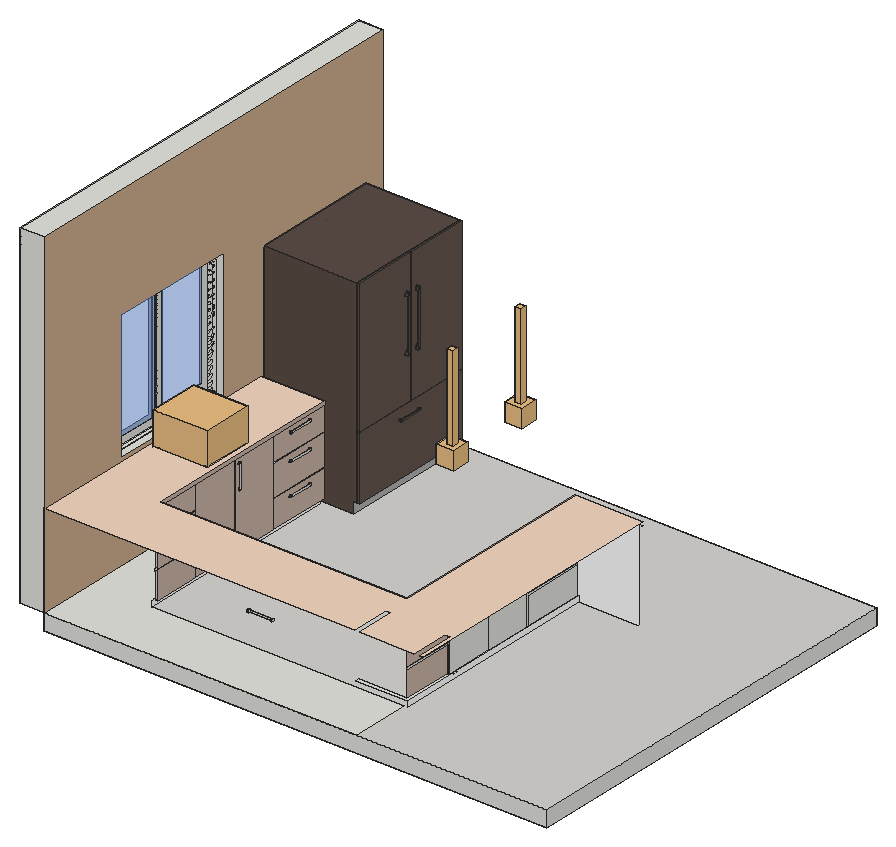
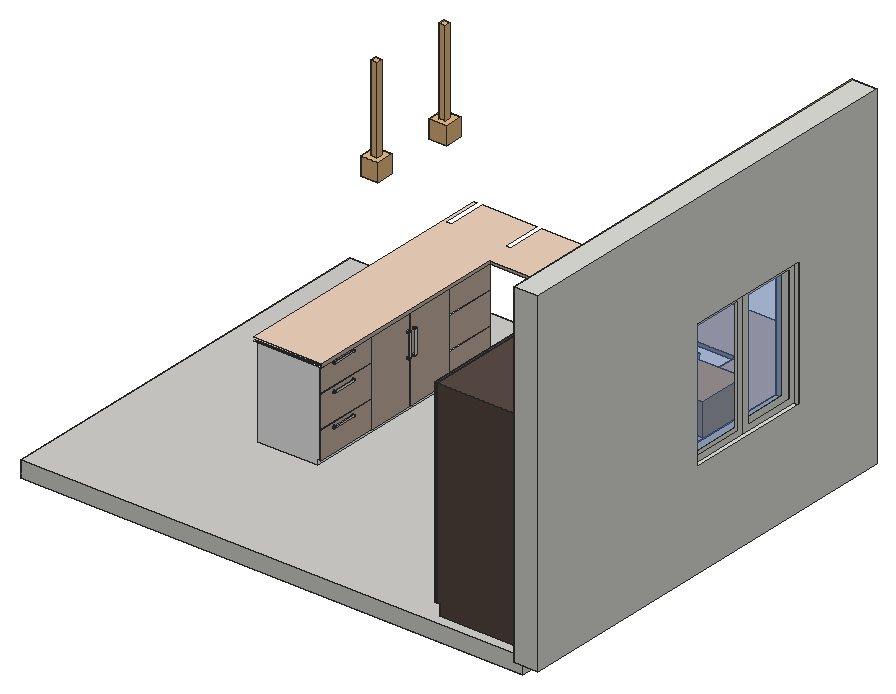
# SketchUp Ruby script. Lengths in inches.
U = 1.inch
M = Sketchup.active_model
def pt(a) = Geom::Point3d.new(a.map { |v| v * U })
def face(e, loops, mat)
  f = e.add_face(loops[0].map { |a| pt(a) })
  loops[1..].each { |l| e.add_face(l.map { |a| pt(a) }).erase! }
  f.material = f.back_material = mat if mat
  f
end
# faces: each face lists its corners as indices into pts; further lists are holes
def faces(e, pts, list, mat = nil) = list.each { |f| face(e, (f[0].is_a?(Array) ? f : [f]).map { |l| l.map { |i| pts[i] } }, mat) }
# xy, xz, yz: faces in a plane at the given z, y or x. An outline is a flat list of corners, or four numbers for a rectangle; further outlines are holes
def ring(l) = l.size == 4 ? [[l[0], l[1]], [l[2], l[1]], [l[2], l[3]], [l[0], l[3]]] : l.each_slice(2).to_a
def flat(e, list, mat, &to3) = list.each { |f| face(e, (f[0].is_a?(Array) ? f : [f]).map { |l| ring(l).map { |u, v| to3.(u, v) } }, mat) }
def xy(e, z, list, mat = nil) = flat(e, list, mat) { |x, y| [x, y, z] }
def xz(e, y, list, mat = nil) = flat(e, list, mat) { |x, z| [x, y, z] }
def yz(e, x, list, mat = nil) = flat(e, list, mat) { |y, z| [x, y, z] }
def lines(e, pts, list) = list.each { |a, b| e.add_line(pt(pts[a]), pt(pts[b])) }
# prism: a flat outline (further loops are holes) pulled along v
def prism(e, loops, v, mat = nil)
  f = face(e, loops, mat); d = Geom::Vector3d.new(v.map { |x| x * U })
  f.pushpull(f.normal.samedirection?(d) ? d.length : -d.length)
end
def box(e, o, s, mat = nil) = prism(e, [[o, [o[0] + s[0], o[1], o[2]], [o[0] + s[0], o[1] + s[1], o[2]], [o[0], o[1] + s[1], o[2]]]], [0, 0, s[2]], mat)
def at(x, y, z, deg = 0) = Geom::Transformation.translation(pt([x, y, z])) * Geom::Transformation.rotation(ORIGIN, Z_AXIS, deg.degrees)
def axes(o, x, y, z) = Geom::Transformation.new([*x, 0, *y, 0, *z, 0, *pt(o).to_a, 1])
def part(name) = M.definitions.add(name)
# library, detail: a bought-in or finely detailed component or shape, given as its bounding box
def library(name, o, s) = part(name).tap { |d| box(d.entities, o, s) }
def detail(e, o, s) = box(e.add_group.entities, o, s)
def put(e, d, t, mat = nil) = e.add_instance(d, t).tap { |i| i.material = mat if mat }
def group(e, t, mat = nil) = e.add_group.tap { |g| g.transformation = t; g.material = mat if mat }.entities
root = M.entities
M.materials.add("2").color = [91, 76, 69]
M.materials.add("Emissive\#2").color = [255, 255, 255]
M.materials.add("Emissive\#3").color = [255, 255, 255]
M.materials.add("[0008_LavenderBlush]").color = [212, 210, 207]
M.materials.add("[Aluminum]").color = [179, 179, 179]
M.materials.add("[Color A01]5").color = [206, 173, 143]
M.materials.add("[Color B01]").color = [102, 86, 78]
M.materials.add("[Color D01]").color = [201, 180, 165]
M.materials.add("[Color D02]").color = [242, 213, 191]
M.materials.add("[Translucent Glass Blue]").color = [100, 149, 237]
M.materials["[Translucent Glass Blue]"].alpha = 0.5
c1 = part("Group\#8")
prism(c1.entities,[[[0.125,0.37,0],[0.125,1.02,0],[0.125,1.04,0],[0.125,1.0625,0.01],[0.125,1.08,0.01],[0.125,1.1,0.02],[0.125,1.12,0.04],[0.125,1.14,0.05],[0.125,1.15,0.07],[0.125,1.16,0.09],[0.125,1.17,0.11],[0.125,1.18,0.125],[0.125,1.1875,0.15],[0.125,1.1875,0.17],[0.125,1.1875,3.72],[0.125,1.18,3.74],[0.125,1.18,3.76],[0.125,1.17,3.78],[0.125,1.16,3.8],[0.125,1.14,3.81],[0.125,1.125,3.83],[0.125,1.11,3.84],[0.125,1.09,3.85],[0.125,1.07,3.86],[0.125,1.05,3.87],[0.125,1.03,3.875],[0.125,1.01,3.875],[0.125,0.37,3.875],[0.125,0.37,3.625],[0.125,0.9375,3.625],[0.125,0.9375,0.25],[0.125,0.37,0.25]]],[-0.125,0,0])
c2 = part("Group\#171")
prism(c2.entities,[[[0,0.37,0],[0,0.37,0.25],[0,0.9375,0.25],[0,0.9375,3.625],[0,0.37,3.625],[0,0.37,3.875],[0,1.01,3.875],[0,1.03,3.875],[0,1.05,3.87],[0,1.07,3.86],[0,1.09,3.85],[0,1.11,3.84],[0,1.125,3.83],[0,1.14,3.81],[0,1.16,3.8],[0,1.17,3.78],[0,1.18,3.76],[0,1.18,3.74],[0,1.1875,3.72],[0,1.1875,0.17],[0,1.1875,0.15],[0,1.18,0.125],[0,1.17,0.11],[0,1.16,0.09],[0,1.15,0.07],[0,1.14,0.05],[0,1.12,0.04],[0,1.1,0.02],[0,1.08,0.01],[0,1.0625,0.01],[0,1.04,0],[0,1.02,0]]],[0.125,0,0])
c3 = library("Pendant light \#2",[-0.17,-0.17,-2.26],[2.36,2.36,34.63])
c4 = library("Sink with faucet",[-0.11,0,0],[20.3,18.9,21.51])
xy(root,6,[[8.9375,9,8.9375,110.3125,31.25,110.3125,31.25,31.3125,125.9375,31.3125,125.9375,9]])
xy(root,6,[[9,111.6875,11.8125,159.6875],[11.8125,111.6875,42.9375,159.6875]],"2")
xy(root,8,[[107.9375,31.3125,107.9375,32.625,125.9375,32.625,125.9375,51.3125,127.25,51.3125,127.25,31.3125],[31.25,32.625,31.9375,50],[31.9375,32.625,32.5625,50],[31.25,50,31.9375,50.5],[31.25,50.5,31.9375,68.5],
  [31.9375,50.5,32.5625,68.5],[126.5625,51.3125,127.25,51.8125],[125.9375,51.8125,126.5625,69.8125],[126.5625,51.8125,127.25,69.8125],[31.25,68.5,31.9375,69],
  [31.25,69,31.9375,86.5],[31.9375,69,32.5625,86.5],[125.9375,69.8125,126.5625,70.3125],[126.5625,69.8125,127.25,111.625],[125.9375,70.3125,126.5625,87.8125],
  [31.25,86.5,31.9375,86.99],[31.25,86.99,31.9375,110.3125],[31.9375,86.99,32.5625,110.3125],[125.9375,87.8125,126.5625,88.3],[125.9375,88.3,126.5625,111.625]])
xy(root,10.07,[[11.8125,111.6875,12.875,135.1875],[42.9375,111.6875,44,135.1875],[44,111.6875,45,159.6875],[11.8125,135.1875,12.875,136.1875],[42.9375,135.1875,44,136.1875],
  [42.9375,136.1875,44,159.6875]],"2")
xy(root,18.125,[[31.9375,32.625,32.5625,50],[31.9375,86.99,32.5625,110.3125],[125.9375,88.3,126.5625,111.625]])
xy(root,18.625,[[31.9375,32.625,32.5625,50],[31.9375,86.99,32.5625,110.3125],[125.9375,88.3,126.5625,111.625]])
xy(root,28.5,[[12.67,58,30.19,58,30.29,58.02,30.39,58.06,30.48,58.1,30.57,58.16,30.64,58.23,30.71,58.31,30.77,58.39,30.81,58.48,30.85,58.58,30.87,58.68,30.875,58.79,30.875,76.11,30.87,76.21,30.85,76.3125,30.81,76.41,30.77,76.5,30.71,76.59,30.57,76.73,30.48,76.79,30.39,76.84,30.29,76.87,30.19,76.89,30.09,76.9,12.76,76.9,12.66,76.89,12.5625,76.87,12.46,76.84,12.37,76.79,12.29,76.73,12.21,76.66,12.14,76.59,12.08,76.5,12.04,76.41,12,76.3125,11.98,76.21,11.98,58.68,12,58.59,12.03,58.5,12.07,58.41,12.12,58.33,12.24,58.19,12.4,58.09,12.49,58.05,12.58,58.02]])
xy(root,30.125,[[31.9375,32.625,32.5625,50],[31.9375,86.99,32.5625,110.3125],[125.9375,88.3,126.5625,111.625]])
xy(root,30.625,[[31.9375,32.625,32.5625,50],[31.9375,86.99,32.5625,110.3125],[125.9375,88.3,126.5625,111.625]])
xy(root,33.92,[[44,111.6875,45,159.6875]],"2")
xy(root,34.38,[[12.875,111.6875,13.875,135.1875],[44,111.6875,45,135.1875],[44,136.1875,45,159.6875]],"2")
xy(root,39.75,[[31.9375,32.625,32.5625,32.75],[31.9375,32.75,32.5625,50],[31.9375,50.5,32.5625,68.5],[125.9375,51.8125,126.5625,69.8125],[31.9375,69,32.5625,86.5],
  [125.9375,70.3125,126.5625,87.8125],[31.9375,86.99,32.5625,110.3125],[125.9375,88.3,126.5625,111.625]])
xy(root,39.75,[[49.9375,32,49.9375,32.625,32.5625,32.625,32.5625,32.75,32.6875,32.75,32.6875,33.25,125.3125,33.25,125.3125,112.25,150.8125,112.25,150.8125,111.625,125.9375,111.625,125.9375,88.3,126.5625,88.3,126.5625,87.8125,125.9375,87.8125,125.9375,70.3125,126.5625,70.3125,126.5625,69.8125,125.9375,69.8125,125.9375,51.8125,126.5625,51.8125,126.5625,51.3125,125.9375,51.3125,125.9375,32.625,107.9375,32.625,107.9375,32,107.4375,32,107.4375,32.625,89.4375,32.625,89.4375,32,88.9375,32,88.9375,32.625,50.4375,32.625,50.4375,32],[32.5625,32.75,32.5625,50,31.9375,50,31.9375,50.5,32.5625,50.5,32.5625,68.5,31.9375,68.5,31.9375,69,32.5625,69,32.5625,86.5,31.9375,86.5,31.9375,86.99,32.5625,86.99,32.5625,110.3125,33.1875,110.3125,33.1875,33.25,32.6875,33.25,32.6875,32.75]],"Emissive\#2")
xy(root,41,[[[8.9375,9,125.3125,9,125.3125,23.51,127.1875,23.51,127.1875,9,147.625,9,147.625,23.51,149.5625,23.51,149.5625,9,150.8125,9,150.8125,112.25,125.3125,112.25,125.3125,33.25,33.1875,33.25,33.1875,110.3125,8.9375,110.3125],[12.67,58,12.58,58.02,12.49,58.05,12.4,58.09,12.24,58.19,12.12,58.33,12.07,58.41,12.03,58.5,12,58.59,11.98,58.68,11.98,76.21,12,76.3125,12.04,76.41,12.08,76.5,12.14,76.59,12.21,76.66,12.29,76.73,12.37,76.79,12.46,76.84,12.5625,76.87,12.66,76.89,12.76,76.9,30.09,76.9,30.19,76.89,30.29,76.87,30.39,76.84,30.48,76.79,30.57,76.73,30.71,76.59,30.77,76.5,30.81,76.41,30.85,76.3125,30.87,76.21,30.875,76.11,30.875,58.79,30.87,58.68,30.85,58.58,30.81,58.48,30.77,58.39,30.71,58.31,30.64,58.23,30.57,58.16,30.48,58.1,30.39,58.06,30.29,58.02,30.19,58]]],"[Color D02]")
xy(root,84,[[9,111.6875,44,159.6875],[44,111.6875,45,135.1875],[44,136.1875,45,159.6875]],"2")
xz(root,33.25,[[33.1875,39.75,125.3125,41]],"[Color D01]")
xz(root,50,[[31.9375,8,32.5625,18.125],[31.9375,18.625,32.5625,28.25],[31.9375,28.25,32.5625,30.125],[31.9375,30.625,32.5625,39.0625],[31.9375,39.0625,32.5625,39.75]])
xz(root,50.5,[[31.9375,8,32.5625,39.75]])
xz(root,51.3125,[[125.9375,8,126.5625,18.125],[125.9375,18.625,126.5625,28.25],[125.9375,28.25,126.5625,30.125],[125.9375,30.625,126.5625,39.0625],[125.9375,39.0625,126.5625,39.75]])
xz(root,51.8125,[[125.9375,8,126.5625,39.75]])
xz(root,58,[[12.67,28.5,12.76,41],[12.76,28.5,30.09,41],[30.09,28.5,30.19,41]])
xz(root,68.5,[[31.9375,8,32.5625,39.75]])
xz(root,69,[[31.9375,8,32.5625,39.75]])
xz(root,69.8125,[[125.9375,8,126.5625,39.75]])
xz(root,70.3125,[[125.9375,8,126.5625,39.75]])
xz(root,76.9,[[12.76,28.5,30.09,41]])
xz(root,86.5,[[31.9375,8,32.5625,39.75]])
xz(root,86.99,[[31.9375,8,32.5625,15.75],[31.9375,15.75,32.5625,16.25],[31.9375,16.25,32.5625,18.125],[31.9375,18.625,32.5625,27.75],[31.9375,27.75,32.5625,28.25],
  [31.9375,28.25,32.5625,30.125],[31.9375,30.625,32.5625,39.75]])
xz(root,87.8125,[[125.9375,8,126.5625,39.75]])
xz(root,88.3,[[125.9375,8,126.5625,15.75],[125.9375,15.75,126.5625,16.25],[125.9375,16.25,126.5625,18.125],[125.9375,18.625,126.5625,27.75],[125.9375,27.75,126.5625,28.25],
  [125.9375,28.25,126.5625,30.125],[125.9375,30.625,126.5625,39.75]])
xz(root,110.3125,[[8.9375,6,8.9375,41,33.1875,41,33.1875,39.75,31.9375,39.75,31.9375,8,31.25,8,31.25,6],[31.9375,8,32.5625,18.125],[31.9375,18.625,32.5625,30.125],[31.9375,30.625,32.5625,39.75]])
xz(root,111.625,[[125.9375,8,126.5625,18.125],[125.9375,18.625,126.5625,30.125],[125.9375,30.625,126.5625,39.75]])
xz(root,111.625,[[127.25,6,127.25,8,126.5625,8,126.5625,39.75,149.5625,39.75,149.5625,6]],"Emissive\#3")
xz(root,111.6875,[[9,6,11.8125,6,11.8125,10.07,12.875,10.07,12.875,33.92,13.875,33.92,13.875,10.07,11.8125,10.07,11.8125,6,42.9375,6,42.9375,10.07,44,10.07,44,84,9,84],[12.875,10.07,13.875,33.92],[44,10.07,45,33.92],[44,34.38,45,84]],"2")
xz(root,135.1875,[[44,34.38,45,84]],"2")
xz(root,136.1875,[[44,34.38,45,84]],"2")
xz(root,159.6875,[[9,6,9,84,44,84,44,10.07,42.9375,10.07,42.9375,6],[44,10.07,45,33.92],[44,34.38,45,84]],"2")
yz(root,8.9375,[[9,6,110.3125,41]])
yz(root,9,[[111.6875,6,159.6875,84]],"2")
yz(root,11.98,[[58.68,28.5,76.11,41],[76.11,28.5,76.21,41]])
yz(root,12.875,[[111.6875,10.07,135.1875,33.92],[135.1875,10.07,136.1875,33.92],[111.6875,33.92,135.1875,34.38],[135.1875,33.92,136.1875,34.38]],"2")
yz(root,30.875,[[58.79,28.5,76.11,41]])
yz(root,31.25,[[31.3125,6,110.3125,8]],"Emissive\#2")
yz(root,31.9375,[[50,8,50.5,8,50.5,39.75,50,39.75,50,30.625,32,30.625,32,30.125,50,30.125,50,18.625,32,18.625,32,18.125,50,18.125],[32.625,8,50,18.125],[50.5,8,68.5,39.75],[68.5,8,69,39.75],[69,8,86.5,39.75],
  [86.5,8,86.99,8,86.99,18.125,110.3125,18.125,110.3125,18.625,86.99,18.625,86.99,30.125,110.3125,30.125,110.3125,30.625,86.99,30.625,86.99,39.75,86.5,39.75],[86.99,8,110.3125,18.125],[32.625,18.625,50,30.125],[86.99,18.625,110.3125,30.125],[32.625,30.625,50,39.75],
  [86.99,30.625,110.3125,39.75]])
yz(root,32.5625,[[32.625,8,50,18.125],[50.5,8,68.5,39.75],[69,8,86.5,39.75],[86.99,8,110.3125,18.125],[32.625,18.625,50,30.125],
  [86.99,18.625,110.3125,30.125],[32.625,30.625,50,39.75],[86.99,30.625,110.3125,39.75]],"[Color D01]")
yz(root,33.1875,[[33.25,39.75,110.3125,41]],"[Color D01]")
yz(root,42.9375,[[111.6875,6,159.6875,10.07]],"[Aluminum]")
yz(root,44,[[111.6875,10.07,135.1875,33.92],[135.1875,10.07,136.1875,33.92],[136.1875,10.07,159.6875,33.92],[111.6875,33.92,135.1875,34.38],[135.1875,33.92,136.1875,34.38],
  [136.1875,33.92,159.6875,34.38],[111.6875,34.38,135.1875,84],[135.1875,34.38,136.1875,84],[136.1875,34.38,159.6875,84]],"2")
yz(root,45,[[111.6875,10.07,159.6875,33.92],[111.6875,34.38,135.1875,84],[136.1875,34.38,159.6875,84]],"[Color B01]")
yz(root,125.3125,[[33.25,39.75,112.25,41]],"[Color D01]")
yz(root,125.9375,[[32.625,8,51.3125,18.125],[51.8125,8,69.8125,39.75],[70.3125,8,87.8125,39.75],[88.3,8,111.625,18.125],[32.625,18.625,51.3125,30.125],
  [88.3,18.625,111.625,30.125],[32.625,30.625,51.3125,39.75],[88.3,30.625,111.625,39.75]],"[Color D01]")
yz(root,126.5625,[[51.3125,8,51.3125,18.125,32,18.125,32,18.625,51.3125,18.625,51.3125,30.125,32,30.125,32,30.625,51.3125,30.625,51.3125,39.75,51.8125,39.75,51.8125,8],[51.8125,8,69.8125,39.75],[69.8125,8,70.3125,39.75],[70.3125,8,87.8125,39.75],[87.8125,8,87.8125,39.75,88.3,39.75,88.3,30.625,111.625,30.625,111.625,30.125,88.3,30.125,88.3,18.625,111.625,18.625,111.625,18.125,88.3,18.125,88.3,8],
  [88.3,8,111.625,18.125],[88.3,18.625,111.625,30.125],[88.3,30.625,111.625,39.75]])
yz(root,127.25,[[31.3125,6,111.625,8]],"Emissive\#2")
p = [[12.4,58.09,41],[12.49,58.05,41],[12.49,58.05,28.5],[12.4,58.09,28.5],[12.58,58.02,41],[12.58,58.02,28.5],
  [12.67,58,41],[12.67,58,28.5],[30.19,58,41],[30.29,58.02,41],[30.29,58.02,28.5],[30.19,58,28.5],
  [30.39,58.06,41],[30.39,58.06,28.5],[12.24,58.19,41],[12.32,58.14,41],[12.32,58.14,28.5],[12.24,58.19,28.5],
  [30.48,58.1,41],[30.48,58.1,28.5],[30.57,58.16,41],[30.57,58.16,28.5],[12.18,58.26,41],[12.18,58.26,28.5],
  [30.64,58.23,41],[30.64,58.23,28.5],[30.71,58.31,41],[30.71,58.31,28.5],[12.12,58.33,41],[12.12,58.33,28.5],
  [12.07,58.41,41],[12.07,58.41,28.5],[30.77,58.39,41],[30.77,58.39,28.5],[12.03,58.5,41],[12.03,58.5,28.5],
  [30.81,58.48,41],[30.81,58.48,28.5],[12,58.59,41],[12,58.59,28.5],[30.85,58.58,41],[30.85,58.58,28.5],
  [11.98,58.68,41],[11.98,58.68,28.5],[30.87,58.68,41],[30.87,58.68,28.5],[30.875,58.79,41],[30.875,58.79,28.5],
  [30.875,76.11,41],[30.87,76.21,41],[30.87,76.21,28.5],[30.875,76.11,28.5],[12,76.3125,41],[11.98,76.21,41],
  [11.98,76.21,28.5],[12,76.3125,28.5],[30.85,76.3125,41],[30.85,76.3125,28.5],[12.04,76.41,41],[12.04,76.41,28.5],
  [30.81,76.41,41],[30.81,76.41,28.5],[12.08,76.5,41],[12.08,76.5,28.5],[30.77,76.5,41],[30.77,76.5,28.5],
  [12.14,76.59,41],[12.14,76.59,28.5],[30.71,76.59,41],[30.71,76.59,28.5],[12.21,76.66,41],[12.21,76.66,28.5],
  [30.64,76.66,41],[30.64,76.66,28.5],[12.29,76.73,41],[12.29,76.73,28.5],[12.37,76.79,41],[12.37,76.79,28.5],
  [30.57,76.73,41],[30.48,76.79,41],[30.48,76.79,28.5],[30.57,76.73,28.5],[12.46,76.84,41],[12.46,76.84,28.5],
  [12.5625,76.87,41],[12.5625,76.87,28.5],[30.39,76.84,41],[30.29,76.87,41],[30.29,76.87,28.5],[30.39,76.84,28.5],
  [12.66,76.89,41],[12.66,76.89,28.5],[12.76,76.9,41],[12.76,76.9,28.5],[30.19,76.89,41],[30.09,76.9,41],
  [30.09,76.9,28.5],[30.19,76.89,28.5],[31.9375,50,39.75],[31.9375,50,40.1875],[126.5625,51.3125,39.75],[126.5625,51.3125,40.1875],
  [126.5625,33.9375,39.75],[13.875,159.6875,34.38],[13.875,136.1875,34.38],[12.875,136.1875,33.92],[12.875,159.6875,33.92],[13.875,135.1875,34.38],
  [13.875,135.1875,84],[12.875,136.1875,34.38],[13.875,111.6875,33.92],[13.875,159.6875,33.92]]
faces(root,p,[[0,1,2,3],[1,4,5,2],[4,6,7,5],[8,9,10,11],[9,12,13,10],[14,15,16,17],[15,0,3,16],[12,18,19,13],
  [18,20,21,19],[22,14,17,23],[20,24,25,21],[24,26,27,25],[28,22,23,29],[30,28,29,31],[26,32,33,27],[34,30,31,35],
  [32,36,37,33],[38,34,35,39],[36,40,41,37],[42,38,39,43],[40,44,45,41],[44,46,47,45],[48,49,50,51],[52,53,54,55],
  [49,56,57,50],[58,52,55,59],[56,60,61,57],[62,58,59,63],[60,64,65,61],[66,62,63,67],[64,68,69,65],[70,66,67,71],
  [68,72,73,69],[74,70,71,75],[76,74,75,77],[78,79,80,81],[72,78,81,73],[82,76,77,83],[84,82,83,85],[86,87,88,89],
  [79,86,89,80],[90,84,85,91],[92,90,91,93],[94,95,96,97],[87,94,97,88]])
lines(root,p,[[98,99],[100,101],[102,100],[103,104],[105,106],[107,108],[104,109],[110,111]])
detail(root,[130.04,41.22,84.29],[6.61,6.58,6.69])
detail(root,[130.91,72.13,85.16],[6.61,6.58,6.7])
put(root,c1,axes([47.77,32.24,27.45],[-4.5235,0,0],[0,1.03829,0],[0,0,2.4525]))
put(root,c1,axes([106.9,32.24,27.45],[-4.5235,0,0],[0,1.03829,0],[0,0,2.4525]))
put(root,c1,axes([109.02,32.24,27.45],[-4.5235,0,0],[0,1.03829,0],[0,0,2.4525]))
put(root,c2,axes([75.47,32.23,16.45],[0,0,-4.5235],[0,1.07125,0],[-2.4525,0,0]))
put(root,c2,axes([75.47,32.23,28.51],[0,0,-4.5235],[0,1.07125,0],[-2.4525,0,0]))
put(root,c2,axes([75.47,32.23,38.32],[0,0,-4.5235],[0,1.07125,0],[-2.4525,0,0]))
put(root,c3,at(132.37,45.47,90.44,-90))
put(root,c4,at(10.68,58,31.63))
put(root,c2,axes([125.9375,69.14,24.73],[0,-4.5235,0],[-1.07125,0,0],[0,0,2.4525]))
put(root,c1,axes([32.2,70.15,28.5],[0,4.5235,0],[1.03829,0,0],[0,0,2.4525]))
put(root,c2,axes([125.9375,71.89,24.73],[0,-4.5235,0],[-1.07125,0,0],[0,0,2.4525]))
put(root,c3,at(133.23,76.39,91.32,-90))
g1 = group(root,at(8.9375,9,0))
xy(g1,0,[[0,0,188.25,154.4375]])
xy(g1,6,[[0,0,188.25,154.4375]],"[0008_LavenderBlush]")
xz(g1,0,[[0,0,188.25,6]])
xz(g1,154.4375,[[0,0,188.25,6]])
yz(g1,0,[[0,0,154.4375,6]])
yz(g1,188.25,[[0,0,154.4375,6]])
g2 = group(root,at(0,9,6))
g3 = group(g2,at(0,84,36))
xy(g3,0,[[0,-47.24,1.57,0],[1.57,-47.24,2.76,-23.62],[3.9375,-47.24,5.91,0],[2.76,-25.98,3.9375,0]])
xy(g3,48,[[0,-47.24,1.57,0],[1.57,-47.24,2.76,-23.62],[2.76,-47.24,3.9375,-25.98],[3.9375,-47.24,3.9375,-25.98,2.76,-25.98,2.76,0,5.91,0,5.91,-47.24]])
xz(g3,-47.24,[[0,0,1.57,48],[1.57,0,2.76,48],[3.9375,0,5.91,48]])
xz(g3,-25.98,[[2.76,0,3.9375,48]])
xz(g3,-23.62,[[1.57,0,2.76,48]])
xz(g3,0,[[0,0,1.57,48],[2.76,0,5.91,48]])
yz(g3,1.57,[[[-47.24,0,-23.62,48],[-45.28,2.18,-25.7,45.82]],[-23.62,0,-23.62,45.82,-21.26,45.82,-21.26,2.18,-1.97,2.18,-1.97,45.82,-23.62,45.82,-23.62,48,0,48,0,0]])
yz(g3,2.76,[[-25.98,0,-23.62,48],[[-23.62,0,0,48],[-21.26,2.62,-2.36,45.38]]])
yz(g3,2.76,[[-21.26,2.62,-2.36,45.38]],"[Translucent Glass Blue]")
yz(g3,3.9375,[[-47.24,0,-25.98,0,-25.98,2.62,-44.88,2.62,-44.88,45.38,-25.98,45.38,-25.98,48,-47.24,48]])
yz(g3,3.9375,[[-44.88,2.62,-25.98,45.38]],"[Translucent Glass Blue]")
g4 = group(g2,at(0,0,0))
xy(g4,0,[[0,0,9,158.625]])
xy(g4,36,[[0,36,4.5,84],[4.5,36,5.4375,84],[5.4375,36,9,84]])
xy(g4,84,[[0,36,4.5,84],[4.5,36,5.4375,84],[5.4375,36,9,84]])
xy(g4,126,[[0,0,9,158.625]])
xz(g4,0,[[0,0,9,126]])
xz(g4,36,[[0,36,4.5,84],[4.5,36,5.4375,84],[5.4375,36,9,84]])
xz(g4,84,[[0,36,4.5,84],[4.5,36,5.4375,84],[5.4375,36,9,84]])
xz(g4,158.625,[[0,0,9,126]])
yz(g4,0,[[[0,0,158.625,126],[36,36,84,84]]])
yz(g4,9,[[[0,0,158.625,126],[36,36,84,84]]],"[Color A01]5")
put(root,c2,axes([32.17,94.1,16.48],[0,0,-4.5235],[1.07125,0,0],[0,2.4525,0]))
put(root,c2,axes([32.17,94.1,28.23],[0,0,-4.5235],[1.07125,0,0],[0,2.4525,0]))
put(root,c2,axes([32.17,94.1,37.85],[0,0,-4.5235],[1.07125,0,0],[0,2.4525,0]))
put(root,c2,axes([126.33,106.4375,17.28],[0,0,-4.5235],[-1.07125,0,0],[0,-2.4525,0]))
put(root,c2,axes([126.33,106.4375,29.16],[0,0,-4.5235],[-1.07125,0,0],[0,-2.4525,0]))
put(root,c2,axes([126.33,106.4375,38.97],[0,0,-4.5235],[-1.07125,0,0],[0,-2.4525,0]))
put(root,c2,axes([13.27,132.1,50.69],[0,4.5235,0],[1.64808,0,0],[0,0,5.45]))
put(root,c2,axes([44.4,133.04,50.69],[0,4.5235,0],[1.64808,0,0],[0,0,5.45]),"2")
g5 = group(root,at(44.4,129.5,30.7),"2")
prism(g5,[[[0.6,0,-0.57],[1.67,0,-0.57],[1.71,0,-0.57],[1.75,0.01,-0.57],[1.78,0.03,-0.57],[1.82,0.06,-0.57],[1.85,0.09,-0.57],[1.875,0.12,-0.57],[1.9,0.16,-0.57],[1.92,0.21,-0.57],[1.9375,0.26,-0.57],[1.95,0.3125,-0.57],[1.95,0.36,-0.57],[1.96,0.42,-0.57],[1.96,9.12,-0.57],[1.95,9.17,-0.57],[1.9375,9.22,-0.57],[1.92,9.27,-0.57],[1.9,9.31,-0.57],[1.88,9.36,-0.57],[1.86,9.39,-0.57],[1.83,9.43,-0.57],[1.8,9.45,-0.57],[1.76,9.48,-0.57],[1.73,9.49,-0.57],[1.69,9.5,-0.57],[1.66,9.5,-0.57],[0.6,9.5,-0.57],[0.6,8.89,-0.57],[1.55,8.89,-0.57],[1.55,0.61,-0.57],[0.6,0.61,-0.57]]],[0,0,0.57])
put(root,c2,axes([13.27,129.5,30.7],[0,0,-4.5235],[1.64808,0,0],[0,2.4525,0]))
put(root,c2,axes([13.27,137.04,50.69],[0,4.5235,0],[1.64808,0,0],[0,0,5.45]))
put(root,c2,axes([44.4,137.79,50.69],[0,4.5235,0],[1.64808,0,0],[0,0,5.45]),"2")
